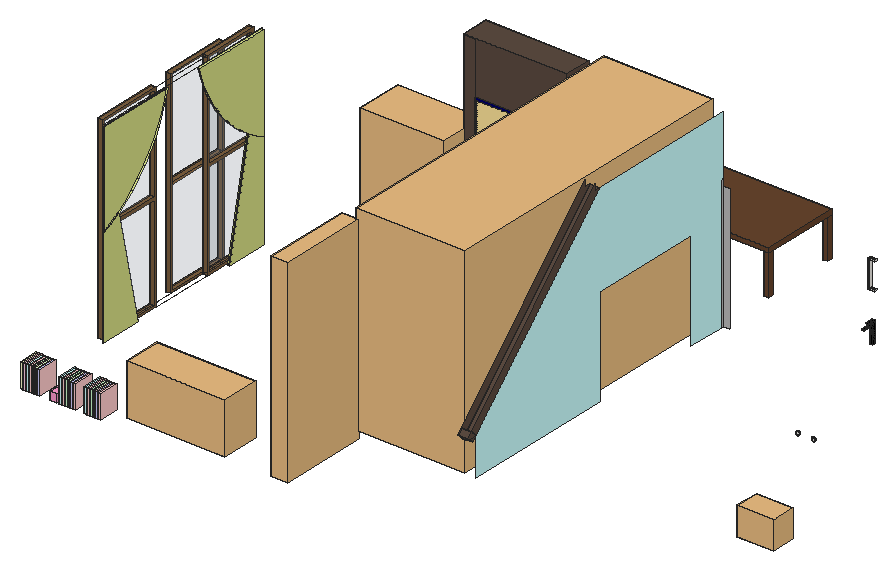
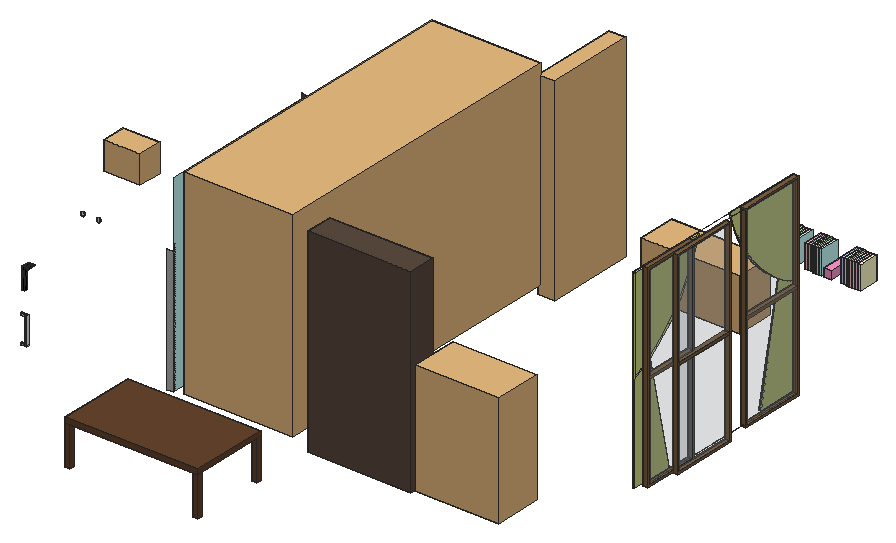
# SketchUp Ruby script. Lengths in inches.
U = 1.inch
M = Sketchup.active_model
def pt(a) = Geom::Point3d.new(a.map { |v| v * U })
def face(e, loops, mat)
  f = e.add_face(loops[0].map { |a| pt(a) })
  loops[1..].each { |l| e.add_face(l.map { |a| pt(a) }).erase! }
  f.material = f.back_material = mat if mat
  f
end
# faces: each face lists its corners as indices into pts; further lists are holes
def faces(e, pts, list, mat = nil) = list.each { |f| face(e, (f[0].is_a?(Array) ? f : [f]).map { |l| l.map { |i| pts[i] } }, mat) }
# xy, xz, yz: faces in a plane at the given z, y or x. An outline is a flat list of corners, or four numbers for a rectangle; further outlines are holes
def ring(l) = l.size == 4 ? [[l[0], l[1]], [l[2], l[1]], [l[2], l[3]], [l[0], l[3]]] : l.each_slice(2).to_a
def flat(e, list, mat, &to3) = list.each { |f| face(e, (f[0].is_a?(Array) ? f : [f]).map { |l| ring(l).map { |u, v| to3.(u, v) } }, mat) }
def xy(e, z, list, mat = nil) = flat(e, list, mat) { |x, y| [x, y, z] }
def xz(e, y, list, mat = nil) = flat(e, list, mat) { |x, z| [x, y, z] }
def yz(e, x, list, mat = nil) = flat(e, list, mat) { |y, z| [x, y, z] }
def lines(e, pts, list) = list.each { |a, b| e.add_line(pt(pts[a]), pt(pts[b])) }
# prism: a flat outline (further loops are holes) pulled along v
def prism(e, loops, v, mat = nil)
  f = face(e, loops, mat); d = Geom::Vector3d.new(v.map { |x| x * U })
  f.pushpull(f.normal.samedirection?(d) ? d.length : -d.length)
end
def box(e, o, s, mat = nil) = prism(e, [[o, [o[0] + s[0], o[1], o[2]], [o[0] + s[0], o[1] + s[1], o[2]], [o[0], o[1] + s[1], o[2]]]], [0, 0, s[2]], mat)
def at(x, y, z, deg = 0) = Geom::Transformation.translation(pt([x, y, z])) * Geom::Transformation.rotation(ORIGIN, Z_AXIS, deg.degrees)
def axes(o, x, y, z) = Geom::Transformation.new([*x, 0, *y, 0, *z, 0, *pt(o).to_a, 1])
def part(name) = M.definitions.add(name)
# library, detail: a bought-in or finely detailed component or shape, given as its bounding box
def library(name, o, s) = part(name).tap { |d| box(d.entities, o, s) }
def detail(e, o, s) = box(e.add_group.entities, o, s)
def put(e, d, t, mat = nil) = e.add_instance(d, t).tap { |i| i.material = mat if mat }
def group(e, t, mat = nil) = e.add_group.tap { |g| g.transformation = t; g.material = mat if mat }.entities
root = M.entities
M.materials.add("A01_Blush_Petal").color = [255, 204, 204]
M.materials.add("Brick_Stack_Bond_2K2").color = [186, 186, 186]
M.materials.add("C01_Vanilla_Cream").color = [255, 230, 206]
M.materials.add("D01_Frost_White").color = [255, 242, 206]
M.materials.add("D02_Buttercup_Glow").color = [255, 229, 155]
M.materials.add("E01_Mint_Frost").color = [255, 255, 204]
M.materials.add("F01_Seafoam_Drift").color = [229, 255, 204]
M.materials.add("G01_Mint_Mist").color = [204, 255, 204]
M.materials.add("Glass_Basic_1").color = [161, 173, 186]
M.materials["Glass_Basic_1"].alpha = 0.25
M.materials.add("H01_Misty_Ice1").color = [204, 255, 255]
M.materials.add("I01_Sky_Frost").color = [204, 204, 255]
M.materials.add("I08_Inkstorm").color = [0, 0, 102]
M.materials.add("L01_Cotton_Candy").color = [255, 204, 229]
M.materials.add("L02_Bubblegum_Pop").color = [255, 153, 204]
M.materials.add("L06_Crimson_Glow").color = [204, 0, 102]
M.materials.add("M02_Ash_Whisper").color = [196, 196, 196]
M.materials.add("M09_Shadow_Night").color = [0, 0, 0]
M.materials.add("Metal_06_1K").color = [238, 236, 231]
M.materials.add("Plywood_01_1K").color = [125, 96, 64]
M.materials.add("Plywood_08_1K").color = [202, 166, 113]
M.materials.add("Wood_Floor_12_1K").color = [92, 75, 65]
M.materials.add("Wood_Grain_45_1K").color = [214, 223, 133]
M.materials.add("Wood_Veneer_15_1K").color = [103, 69, 45]
c1 = part("Group\#83")
xy(c1.entities,0,[[0,-12,1.73,0]])
xy(c1.entities,14.9,[[0,-12,1.73,0]])
xz(c1.entities,-12,[[0,0,1.73,14.9]],"E01_Mint_Frost")
xz(c1.entities,0,[[0,0,1.73,14.9]])
yz(c1.entities,0,[[-12,0,0,14.9]])
yz(c1.entities,1.73,[[-12,0,0,14.9]],"A01_Blush_Petal")
c2 = part("Group\#71")
xy(c2.entities,0,[[0,-12,1.73,0]])
xy(c2.entities,14.9,[[0,-12,1.73,0]])
xz(c2.entities,-12,[[0,0,1.73,14.9]],"F01_Seafoam_Drift")
xz(c2.entities,0,[[0,0,1.73,14.9]])
yz(c2.entities,0,[[-12,0,0,14.9]])
yz(c2.entities,1.73,[[-12,0,0,14.9]],"A01_Blush_Petal")
c3 = part("Group\#63")
xy(c3.entities,0,[[0,-12,1.73,0]])
xy(c3.entities,14.9,[[0,-12,1.73,0]])
xz(c3.entities,-12,[[0,0,1.73,14.9]],"G01_Mint_Mist")
xz(c3.entities,0,[[0,0,1.73,14.9]])
yz(c3.entities,0,[[-12,0,0,14.9]])
yz(c3.entities,1.73,[[-12,0,0,14.9]],"A01_Blush_Petal")
c4 = part("Group\#69")
xy(c4.entities,0,[[0,-12,1.73,0]])
xy(c4.entities,14.9,[[0,-12,1.73,0]])
xz(c4.entities,-12,[[0,0,1.73,14.9]],"H01_Misty_Ice1")
xz(c4.entities,0,[[0,0,1.73,14.9]])
yz(c4.entities,0,[[-12,0,0,14.9]])
yz(c4.entities,1.73,[[-12,0,0,14.9]],"A01_Blush_Petal")
c5 = part("Group\#66")
xy(c5.entities,0,[[0,-12,1.73,0]])
xy(c5.entities,14.9,[[0,-12,1.73,0]],"L01_Cotton_Candy")
xz(c5.entities,-12,[[0,0,1.73,14.9]],"L01_Cotton_Candy")
xz(c5.entities,0,[[0,0,1.73,14.9]])
yz(c5.entities,0,[[-12,0,0,14.9]])
yz(c5.entities,1.73,[[-12,0,0,14.9]],"A01_Blush_Petal")
c6 = part("Group\#84")
xy(c6.entities,0,[[0,-12,1.73,0]])
xy(c6.entities,14.9,[[0,-12,1.73,0]])
xz(c6.entities,-12,[[0,0,1.73,14.9]],"A01_Blush_Petal")
xz(c6.entities,0,[[0,0,1.73,14.9]])
yz(c6.entities,0,[[-12,0,0,14.9]])
yz(c6.entities,1.73,[[-12,0,0,14.9]],"A01_Blush_Petal")
c7 = part("Group\#85")
xy(c7.entities,0,[[0,-12,1.73,0]])
xy(c7.entities,14.9,[[0,-12,1.73,0]])
xz(c7.entities,-12,[[0,0,1.73,14.9]],"I01_Sky_Frost")
xz(c7.entities,0,[[0,0,1.73,14.9]])
yz(c7.entities,0,[[-12,0,0,14.9]])
yz(c7.entities,1.73,[[-12,0,0,14.9]],"A01_Blush_Petal")
c8 = library("Group\#128",[0,0,0],[52.625,19.3125,31.0625])
c9 = library("Decorative Goods 012 Cats",[-6.85,-2.23,0],[13.52,4.53,13.84])
c10 = library("Group\#159",[-9,0,0],[10,53.625,119])
c11 = library("Toilet 005",[-7.26,-21.97,0],[14.52,21.97,16.93])
c12 = library("Group\#6",[0,-1,0],[66,187.375,120])
c13 = part("Group\#178")
prism(c13.entities,[[[0.04,0,1.49],[0.16,0,1.78],[0.35,0,2.03],[0.59,0,2.22],[0.88,0,2.33],[1.1875,0,2.375],[1.49,0,2.33],[1.78,0,2.22],[2.03,0,2.03],[2.22,0,1.78],[2.33,0,1.49],[2.375,0,1.1875],[2.33,0,0.88],[2.22,0,0.59],[2.03,0,0.35],[1.78,0,0.16],[1.49,0,0.04],[1.1875,0,0],[0.88,0,0.04],[0.59,0,0.16],[0.35,0,0.35],[0.16,0,0.59],[0.04,0,0.88],[0,0,1.1875]]],[0,-0.25,0],"Metal_06_1K")
c14 = library("Group\#137",[-1.2,-1.5625,0],[50.9,29.0625,67.875])
c15 = part("Group\#194")
prism(c15.entities,[[[1.51,0.03,0],[1.1875,0,0],[0.87,0.06,0],[0.57,0.2,0],[0.32,0.41,0],[0.14,0.68,0],[0.03,0.98,0],[0,1.31,0],[0.06,1.63,0],[0.2,1.93,0],[0.41,2.17,0],[0.68,2.36,0],[0.98,2.47,0],[1.31,2.5,0],[1.63,2.4375,0],[1.93,2.3,0],[2.17,2.09,0],[2.36,1.82,0],[2.47,1.51,0],[2.5,1.1875,0],[2.4375,0.87,0],[2.3,0.57,0],[2.09,0.32,0],[1.82,0.14,0]]],[0,0,0.25],"Metal_06_1K")
c16 = part("Faucet 017")
xy(c16.entities,0,[[-0.79,-0.79,-0.79,0.79,0.79,-0.79],[0.79,-0.79,-0.79,0.79,0.79,0.79]],"M09_Shadow_Night")
xy(c16.entities,10.22,[[-0.79,-7.09,-0.79,-0.79,0.79,-7.09],[0.79,-7.09,-0.79,-0.79,0.79,-0.79]],"M09_Shadow_Night")
xy(c16.entities,10.73,[[-0.79,-7.09,0.79,-7.09,-0.79,-0.79],[0.79,-7.09,0.79,-0.79,-0.79,-0.79]],"M09_Shadow_Night")
xy(c16.entities,12.44,[[-0.79,-3.9375,-0.79,-0.79,0.79,-3.9375],[0.79,-3.9375,-0.79,-0.79,0.79,-0.79]],"M09_Shadow_Night")
xy(c16.entities,12.83,[[-0.79,-3.9375,0.79,-3.9375,-0.79,0.79],[0.79,-3.9375,0.79,0.79,-0.79,0.79]],"M09_Shadow_Night")
xz(c16.entities,-7.09,[[-0.79,10.22,0.79,10.22,-0.79,10.73],[0.79,10.22,0.79,10.73,-0.79,10.73]],"M09_Shadow_Night")
xz(c16.entities,-3.9375,[[-0.79,12.44,0.79,12.44,0.79,12.83],[-0.79,12.44,0.79,12.83,-0.79,12.83]],"M09_Shadow_Night")
xz(c16.entities,-0.79,[[-0.79,0,0.79,0,0.79,10.22],[-0.79,0,0.79,10.22,-0.79,10.22],[-0.79,10.73,0.79,10.73,-0.79,12.44],[0.79,10.73,0.79,12.44,-0.79,12.44]],"M09_Shadow_Night")
xz(c16.entities,0.79,[[-0.79,0,-0.79,12.83,0.79,0],[0.79,0,-0.79,12.83,0.79,12.83]],"M09_Shadow_Night")
yz(c16.entities,-0.79,[[-0.79,0,-0.79,10.22,0.79,0],[0.79,0,-0.79,10.22,0.79,12.83],[-0.79,10.22,-7.09,10.73,-0.79,10.73],[-7.09,10.22,-7.09,10.73,-0.79,10.22],[-0.79,10.22,-0.79,10.73,0.79,12.83],
  [-0.79,10.73,-0.79,12.44,0.79,12.83],[-0.79,12.44,-3.9375,12.83,0.79,12.83],[-3.9375,12.44,-3.9375,12.83,-0.79,12.44]],"M09_Shadow_Night")
yz(c16.entities,0.79,[[-0.79,0,0.79,0,-0.79,10.22],[0.79,0,0.79,12.83,-0.79,10.22],[-7.09,10.22,-0.79,10.22,-0.79,10.73],[-7.09,10.22,-0.79,10.73,-7.09,10.73],[-0.79,10.22,0.79,12.83,-0.79,10.73],
  [-0.79,10.73,0.79,12.83,-0.79,12.44],[-0.79,12.44,0.79,12.83,-3.9375,12.83],[-3.9375,12.44,-0.79,12.44,-3.9375,12.83]],"M09_Shadow_Night")
c17 = part("Group\#214")
xy(c17.entities,0,[[0.35,-15.79,1.75,-15.1],[0.35,0,1.75,1.15]],"Metal_06_1K")
xy(c17.entities,2.8125,[[0.35,-15.79,1.75,-15.1],[0.35,-15.1,1.75,0],[0.35,0,1.75,1.15]],"Metal_06_1K")
xy(c17.entities,3.8125,[[0.35,-15.79,1.75,-15.1],[0.35,-15.1,1.75,1.15]],"Metal_06_1K")
xz(c17.entities,-15.79,[[0.35,0,1.75,2.8125],[0.35,2.8125,1.75,3.8125]],"Metal_06_1K")
xz(c17.entities,-15.1,[[0.35,0,1.75,2.8125],[0.35,2.8125,1.75,3.8125]],"Metal_06_1K")
xz(c17.entities,0,[[0.35,0,1.75,2.8125]],"Metal_06_1K")
xz(c17.entities,1.15,[[0.35,0,1.75,2.8125],[0.35,2.8125,1.75,3.8125]],"Metal_06_1K")
yz(c17.entities,0.35,[[-15.79,0,-15.1,2.8125],[0,0,1.15,2.8125],[-15.79,2.8125,-15.1,3.8125],[-15.1,2.8125,1.15,3.8125]],"Metal_06_1K")
yz(c17.entities,1.75,[[-15.79,0,-15.1,2.8125],[0,0,1.15,2.8125],[-15.79,2.8125,-15.1,3.8125],[-15.1,2.8125,1.15,3.8125]],"Metal_06_1K")
c18 = part("Group\#255")
box(c18.entities,[0,0,0],[3,3,24],"Wood_Veneer_15_1K")
xy(root,45.8125,[[1876.75,435.3125,1882.75,440.3125]],"Wood_Floor_12_1K")
xz(root,626.6875,[[1882.75,23,1886.75,99]],"Brick_Stack_Bond_2K2")
yz(root,1876.75,[[437.79,43.29,435.3125,45.77,435.3125,45.8125,440.3125,45.8125],[435.3125,45.77,434.26,46.83,436.78,49.35,440.3125,45.8125,435.3125,45.8125],[440.3125,45.8125,436.78,49.35,529.96,142.54,529.96,139,533.5,139]],"Wood_Floor_12_1K")
yz(root,1882.75,[[625.625,23,626.6875,103]],"Brick_Stack_Bond_2K2")
yz(root,1882.75,[[440.3125,23,440.3125,45.8125,533.5,139,626.6875,139,626.6875,103,625.625,103,625.625,23,602.25,23,602.25,82.875,533.5,82.875,533.5,23]],"H01_Misty_Ice1")
yz(root,1882.75,[[437.79,43.29,440.3125,45.8125,435.3125,45.8125,435.3125,45.77],[435.3125,45.77,435.3125,45.8125,440.3125,45.8125,436.78,49.35,434.26,46.83],[440.3125,45.8125,533.5,139,529.96,139,529.96,142.54,436.78,49.35]],"Wood_Floor_12_1K")
p = [[1876.75,437.79,43.29],[1882.75,437.79,43.29],[1882.75,435.3125,45.77],[1882.75,434.26,46.83],[1876.75,434.26,46.83],[1876.75,435.3125,45.77],
  [1876.75,440.3125,45.8125],[1882.75,440.3125,45.8125],[1876.75,436.78,49.35],[1882.75,436.78,49.35],[1882.75,533.5,139],[1876.75,533.5,139]]
faces(root,p,[[0,1,2,3,4,5],[6,7,1,0],[7,6,8,9],[10,7,6,11],[9,8,4,3]],"Wood_Floor_12_1K")
put(root,c1,axes([1675.81,366.75,36.28],[1,0,0],[0,1,0],[0,0,0.96]),"E01_Mint_Frost")
put(root,c2,axes([1684.25,366.75,36.28],[1,0,0],[0,1,0],[0,0,0.96]),"F01_Seafoam_Drift")
put(root,c3,axes([1682.56,366.75,36.28],[1,0,0],[0,1,0],[0,0,0.96]),"G01_Mint_Mist")
put(root,c4,axes([1679.19,366.75,36.28],[1,0,0],[0,1,0],[0,0,0.96]),"H01_Misty_Ice1")
put(root,c5,axes([1677.5,366.75,36.28],[1,0,0],[0,1,0],[0,0,0.96]),"L01_Cotton_Candy")
put(root,c6,axes([1680.88,366.75,36.28],[1,0,0],[0,1,0],[0,0,0.96]),"A01_Blush_Petal")
put(root,c7,axes([1685.98,366.75,36.28],[1,0,0],[0,1,0],[0,0,0.96]),"I01_Sky_Frost")
put(root,c6,axes([1707.63,366.75,36.28],[1,0,0],[0,1,0],[0,0,0.96]),"A01_Blush_Petal")
put(root,c6,axes([1700.88,366.75,36.28],[1,0,0],[0,1,0],[0,0,0.96]),"A01_Blush_Petal")
put(root,c3,axes([1702.56,366.75,36.28],[1,0,0],[0,1,0],[0,0,0.96]),"G01_Mint_Mist")
put(root,c2,axes([1704.25,366.75,36.28],[1,0,0],[0,1,0],[0,0,0.96]),"F01_Seafoam_Drift")
put(root,c4,axes([1699.19,366.75,36.28],[1,0,0],[0,1,0],[0,0,0.96]),"H01_Misty_Ice1")
put(root,c7,axes([1705.98,366.75,36.28],[1,0,0],[0,1,0],[0,0,0.96]),"I01_Sky_Frost")
g1 = group(root,at(1719.37,366.75,36.28),"F01_Seafoam_Drift")
xy(g1,0,[[0,-12,1.73,0]])
xy(g1,14.31,[[0,-12,1.73,0]])
xz(g1,-12,[[0,0,1.73,14.31]],"F01_Seafoam_Drift")
xz(g1,0,[[0,0,1.73,14.31]])
yz(g1,0,[[-12,0,0,14.31]])
yz(g1,1.73,[[-12,0,0,14.31]],"A01_Blush_Petal")
g2 = group(root,at(1721.09,366.75,36.28),"I01_Sky_Frost")
xy(g2,0,[[0,-12,1.73,0]])
xy(g2,14.31,[[0,-12,1.73,0]])
xz(g2,-12,[[0,0,1.73,14.31]],"I01_Sky_Frost")
xz(g2,0,[[0,0,1.73,14.31]])
yz(g2,0,[[-12,0,0,14.31]])
yz(g2,1.73,[[-12,0,0,14.31]],"A01_Blush_Petal")
put(root,c4,axes([1714.3,366.75,36.28],[1,0,0],[0,1,0],[0,0,0.96]),"H01_Misty_Ice1")
put(root,c6,axes([1722.74,366.75,36.28],[1,0,0],[0,1,0],[0,0,0.96]),"A01_Blush_Petal")
put(root,c6,axes([1715.99,366.75,36.28],[1,0,0],[0,1,0],[0,0,0.96]),"A01_Blush_Petal")
put(root,c3,axes([1717.68,366.75,36.28],[1,0,0],[0,1,0],[0,0,0.96]),"G01_Mint_Mist")
g3 = group(root,at(1693.39,366.75,36.28),"L06_Crimson_Glow")
box(g3,[0,-12,0],[4.76,12,4.58],"L02_Bubblegum_Pop")
put(root,c8,axes([1713.84,387.62,19],[1.13,0,0],[0,1.18,0],[0,0,1]),"Plywood_08_1K")
put(root,c9,axes([1731.8125,405.98,36.22],[1,0,0],[0,1,0],[0,0,0.85127]),"C01_Vanilla_Cream")
put(root,c10,at(1810.75,386.6875,19))
put(root,c11,at(2038.75,477.0625,25.33,-90),"M02_Ash_Whisper")
g4 = group(root,at(1654.74,439.7,19),"D01_Frost_White")
yz(g4,0,[[0.98,1.18,39.33,117.82],[80.04,1.18,112.78,117.62]],"Glass_Basic_1")
p = [[1.5,112.78,117.82],[1.5,0.98,117.82],[1.5,0.98,1.18],[1.5,112.78,1.18],[0,78.99,59.78],[0,78.99,58.5]]
lines(g4,p,[[0,1],[1,2],[3,0],[4,5],[2,3]])
g5 = group(g4,at(0,114.03,0))
prism(g5,[[[0,0,0],[0,-35.04,0],[0,-35.04,1.18],[0,-35.04,117.62],[0,-35.04,119],[0,0,119]],[[0,-33.99,117.62],[0,-33.99,59.78],[0,-1.25,59.78],[0,-1.25,117.62]],[[0,-1.25,1.18],[0,-1.25,58.5],[0,-33.99,58.5],[0,-33.99,1.18]]],[3.01,0,0],"Plywood_01_1K")
prism(g5,[[[3.01,-73.83,1.18],[3.01,-73.83,117.62],[3.01,-73.83,119],[3.01,-114.03,119],[3.01,-114.03,0],[3.01,-73.83,0]],[[3.01,-74.71,59.78],[3.01,-113.06,59.78],[3.01,-113.06,117.82],[3.01,-74.71,117.82]],[[3.01,-113.06,1.18],[3.01,-113.06,58.5],[3.01,-74.71,58.5],[3.01,-74.71,1.18]]],[-3.01,0,0],"Plywood_01_1K")
p = [[3.01,-35.04,0],[3.01,-73.83,0]]
lines(g5,p,[[0,1]])
g6 = group(root,at(1659.42,437.09,19),"D01_Frost_White")
p = [[0,0,117.72],[0,120.94,117.72],[0,48.07,116.76],[0,48.12,116.92]]
lines(g6,p,[[0,1],[2,3]])
g7 = group(g6,at(1.11,-0.03,59.1))
xy(g7,-58.86,[[-1,0,0,25.61]],"Wood_Grain_45_1K")
xy(g7,57.9,[[-1,0,0,48.07]],"Wood_Grain_45_1K")
xz(g7,0,[[-1,-58.86,0,0],[-1,0,0,57.9]],"Wood_Grain_45_1K")
yz(g7,-1,[[0,-58.86,0,0,5.77,2.97,11.31,6.35,25.61,-58.86],[0,0,5.77,2.97,11.31,6.35,16.59,10.14,21.57,14.29,26.23,18.81,30.56,23.65,34.51,28.79,38.08,34.22,41.24,39.89,43.98,45.77,46.27,51.84,48.07,57.9,0,57.9]],"Wood_Grain_45_1K")
yz(g7,0,[[0,-58.86,25.61,-58.86,11.31,6.35,5.77,2.97,0,0]],"Wood_Grain_45_1K")
p = [[0,11.31,6.35],[0,25.61,-58.86],[-1,25.61,-58.86],[-1,11.31,6.35],[0,16.59,10.14],[-1,16.59,10.14],
  [0,21.57,14.29],[-1,21.57,14.29],[0,26.23,18.81],[-1,26.23,18.81],[0,30.56,23.65],[-1,30.56,23.65],
  [0,34.51,28.79],[-1,34.51,28.79],[0,38.08,34.22],[-1,38.08,34.22],[0,41.24,39.89],[-1,41.24,39.89],
  [0,43.98,45.77],[-1,43.98,45.77],[0,46.27,51.84],[-1,46.27,51.84],[0,48.07,57.9],[-1,48.07,57.9],
  [0,5.77,2.97],[-1,5.77,2.97]]
faces(g7,p,[[0,1,2,3],[0,4,5,3],[4,6,7,5],[6,8,9,7],[8,10,11,9],[10,12,13,11],[12,14,15,13],[14,16,17,15],
  [16,18,19,17],[18,20,21,19],[20,22,23,21]],"Wood_Grain_45_1K")
lines(g7,p,[[24,25]])
g8 = group(g6,at(-0.12,120.72,59.01))
xy(g8,-58.86,[[0,-25.61,1,0]],"Wood_Grain_45_1K")
xy(g8,57.9,[[0,-48.07,1,0]],"Wood_Grain_45_1K")
xz(g8,0,[[0,-58.86,1,0],[0,0,1,57.9]],"Wood_Grain_45_1K")
yz(g8,0,[[-25.61,-58.86,-11.31,6.35,-5.77,2.97,0,0,0,-58.86]],"Wood_Grain_45_1K")
yz(g8,1,[[-25.61,-58.86,0,-58.86,0,0,-5.77,2.97,-11.31,6.35],[0,0,-5.77,2.97,-11.31,6.35,-16.59,10.14,-21.57,14.29,-26.23,18.81,-30.56,23.65,-34.51,28.79,-38.08,34.22,-41.24,39.89,-43.98,45.77,-46.27,51.84,-48.07,57.9,0,57.9]],"Wood_Grain_45_1K")
p = [[0,-11.31,6.35],[0,-25.61,-58.86],[1,-25.61,-58.86],[1,-11.31,6.35],[0,-16.59,10.14],[1,-16.59,10.14],
  [0,-21.57,14.29],[1,-21.57,14.29],[0,-26.23,18.81],[1,-26.23,18.81],[0,-30.56,23.65],[1,-30.56,23.65],
  [0,-34.51,28.79],[1,-34.51,28.79],[0,-38.08,34.22],[1,-38.08,34.22],[0,-41.24,39.89],[1,-41.24,39.89],
  [0,-43.98,45.77],[1,-43.98,45.77],[0,-46.27,51.84],[1,-46.27,51.84],[0,-48.07,57.9],[1,-48.07,57.9],
  [0,-5.77,2.97],[1,-5.77,2.97]]
faces(g8,p,[[0,1,2,3],[0,4,5,3],[4,6,7,5],[6,8,9,7],[8,10,11,9],[10,12,13,11],[12,14,15,13],[14,16,17,15],
  [16,18,19,17],[18,20,21,19],[20,22,23,21]],"Wood_Grain_45_1K")
lines(g8,p,[[24,25]])
g9 = group(root,at(1654.74,494.39,19),"D01_Frost_White")
xy(g9,0,[[-2.8125,0,0,40.2]],"Plywood_01_1K")
xy(g9,0.88,[[-2.8125,0.88,0,39.33]],"Plywood_01_1K")
xy(g9,58.5,[[-2.8125,0.98,0,39.33]],"Plywood_01_1K")
xy(g9,59.78,[[-2.8125,0.98,0,39.33]],"Plywood_01_1K")
xy(g9,118.12,[[-2.8125,0.88,0,39.33]],"Plywood_01_1K")
xy(g9,119,[[-2.8125,0,0,40.2]],"Plywood_01_1K")
xz(g9,0,[[-2.8125,0,0,119]],"Plywood_01_1K")
xz(g9,0.88,[[-2.8125,0.88,0,118.12]],"Plywood_01_1K")
xz(g9,0.98,[[-2.8125,58.5,0,59.78]],"Plywood_01_1K")
xz(g9,39.33,[[-2.8125,0.88,0,58.5],[-2.8125,58.5,0,59.78],[-2.8125,59.78,0,118.12]],"Plywood_01_1K")
xz(g9,40.2,[[-2.8125,0,0,119]],"Plywood_01_1K")
yz(g9,-2.8125,[[0.88,0.88,0.88,118.12,39.33,118.12,39.33,59.78,0.98,59.78,0.98,58.5,39.33,58.5,39.33,0.88]],"Glass_Basic_1")
yz(g9,-2.8125,[[[0,0,40.2,119],[0.88,0.88,39.33,118.12]],[0.98,58.5,39.33,59.78]],"Plywood_01_1K")
yz(g9,0,[[[0,0,40.2,119],[0.88,0.88,39.33,118.12]]],"Plywood_01_1K")
put(root,c12,at(1810.75,440.3125,24),"Plywood_01_1K")
put(root,c13,at(1992.91,544.25,39.49),"M02_Ash_Whisper")
put(root,c13,at(2002.35,544.25,39.49),"M02_Ash_Whisper")
put(root,c14,at(1689.6,596.64,19),"D01_Frost_White")
g10 = group(root,at(1745.46,610.11,22.92),"D01_Frost_White")
xy(g10,0.375,[[0.375,0,55.54,2]],"I08_Inkstorm")
xy(g10,83.625,[[0.375,0,55.54,2]],"I08_Inkstorm")
xz(g10,0,[[2,2,26.96,42],[28.96,2,53.92,42]])
xz(g10,0,[[2,42,26.96,82],[28.96,42,53.92,82]],"D02_Buttercup_Glow")
xz(g10,0,[[[0.375,0.375,55.54,83.625],[28.96,2,53.92,82],[2,2,26.96,82]]],"I08_Inkstorm")
xz(g10,2,[[[0,0,55.92,84],[0.375,0.375,55.54,83.625]]])
yz(g10,0.375,[[0,0.375,2,83.625]],"I08_Inkstorm")
yz(g10,55.54,[[0,0.375,2,83.625]],"I08_Inkstorm")
put(g10,c15,axes([22.15,0,42.88],[1,0,0],[0,0,1],[0,-1,0]))
put(g10,c15,axes([31.46,0,42.88],[1,0,0],[0,0,1],[0,-1,0]))
g11 = group(root,at(1733.85,610.11,19),"D01_Frost_White")
xy(g11,0,[[5.45,0,67.9,16.58]],"Wood_Floor_12_1K")
xy(g11,4.29,[[11.98,0,67.35,11.25]],"Wood_Floor_12_1K")
xy(g11,87.55,[[11.98,0,67.35,11.25]],"Wood_Floor_12_1K")
xy(g11,119.5,[[5.45,0,67.9,16.58]],"Wood_Floor_12_1K")
xz(g11,0,[[5.45,0,11.98,119],[11.98,0,67.9,4.29],[67.35,4.29,67.9,4.29,67.9,119.5,5.45,119.5,5.45,119,11.98,119,11.98,87.55,67.35,87.55]],"Wood_Floor_12_1K")
xz(g11,11.25,[[11.98,4.29,67.35,87.55]],"Wood_Floor_12_1K")
xz(g11,16.58,[[5.45,0,67.9,119.5]],"Wood_Floor_12_1K")
yz(g11,5.45,[[0,0,16.58,119.5]],"Wood_Floor_12_1K")
yz(g11,11.98,[[0,4.29,11.25,87.55]],"Wood_Floor_12_1K")
yz(g11,67.35,[[0,4.29,11.25,87.55]],"Wood_Floor_12_1K")
yz(g11,67.9,[[0,0,16.58,119.5]],"Wood_Floor_12_1K")
put(root,c16,at(1973.58,625.9,46.04),"M02_Ash_Whisper")
put(root,c17,axes([1942.625,667.97,61.49],[0,-1,0],[0,0,1],[-1,0,0]),"M02_Ash_Whisper")
g12 = group(root,at(1799.85,664.85,18),"M02_Ash_Whisper")
put(g12,c18,at(77.0625,44.5,3))
put(g12,c18,at(0,44.5,3))
g13 = group(g12,at(0,0,0))
g14 = group(g13,at(0,0,27))
box(g14,[0,0,0],[80.0625,47.5,3],"Wood_Veneer_15_1K")
g15 = group(g12,at(0,0,3))
box(g15,[0,0,0],[3,3,24],"Wood_Veneer_15_1K")
put(g12,c18,at(77.0625,0,3))
